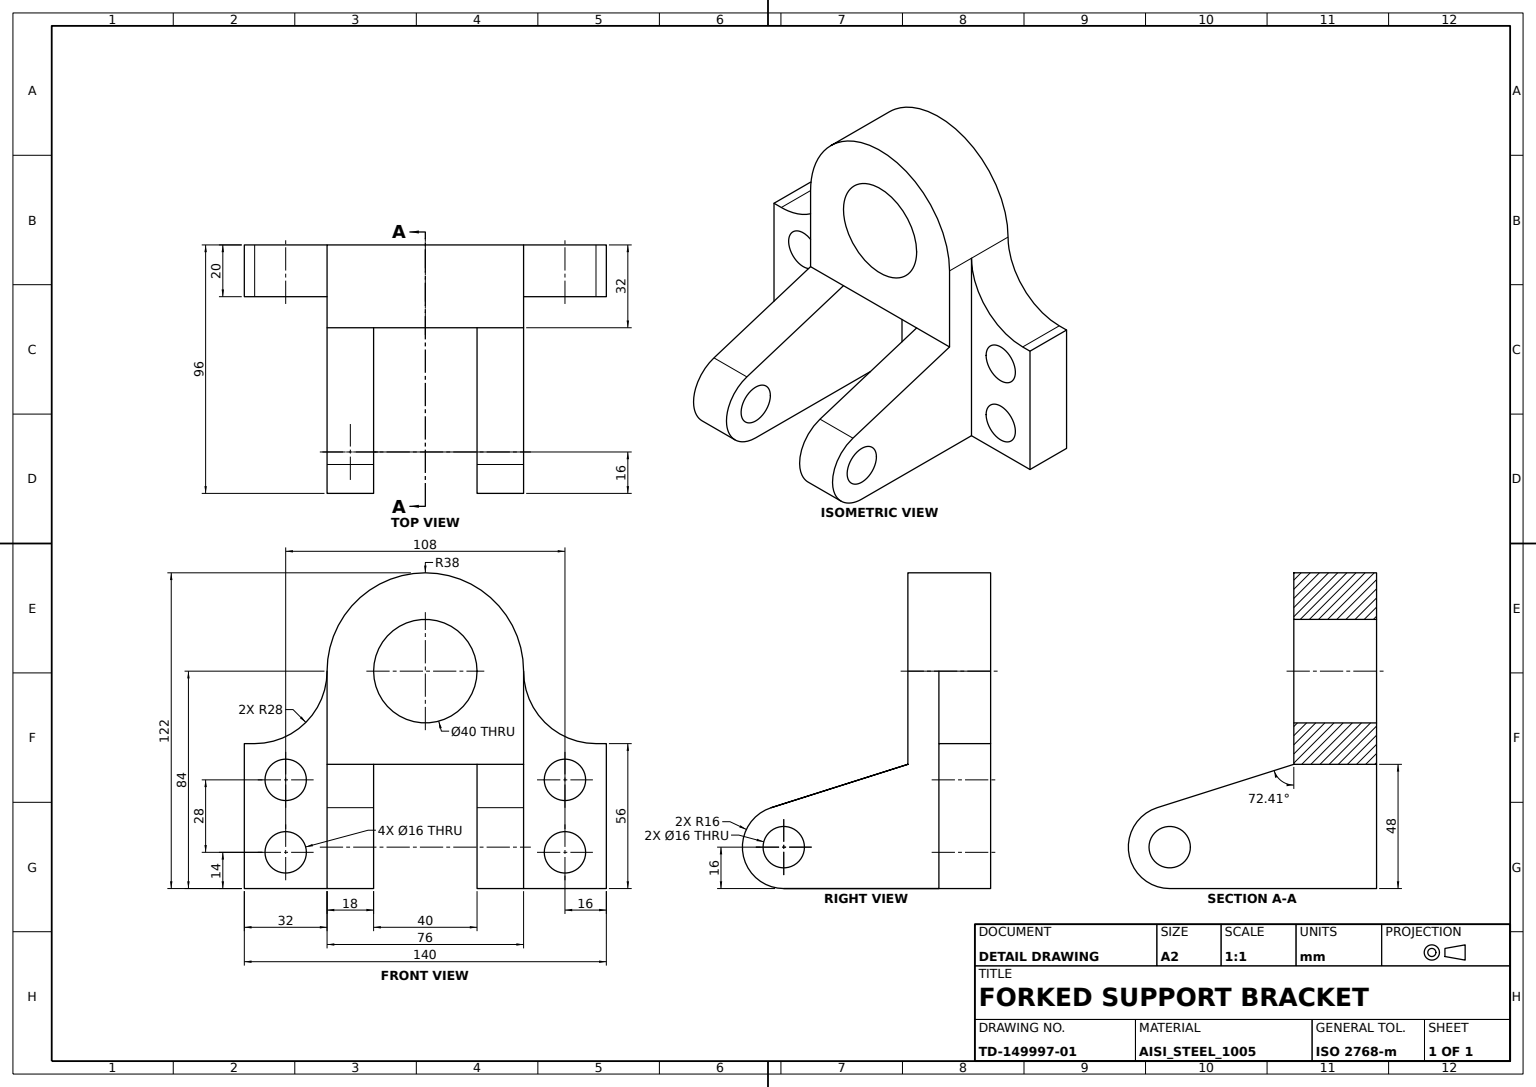
ISO-10303-21;
HEADER;
FILE_DESCRIPTION((''),'2;1');
FILE_NAME('','',(''),(''),'','','');
FILE_SCHEMA(('AUTOMOTIVE_DESIGN'));
ENDSEC;
DATA;
#1=APPLICATION_CONTEXT('');
#2=PRODUCT_CONTEXT('',#1,'mechanical');
#3=PRODUCT('','','',(#2));
#4=PRODUCT_DEFINITION_FORMATION('','',#3);
#5=PRODUCT_DEFINITION_CONTEXT('',#1,'design');
#6=PRODUCT_DEFINITION('','',#4,#5);
#7=PRODUCT_DEFINITION_SHAPE('','',#6);
#8=(LENGTH_UNIT()NAMED_UNIT(*)SI_UNIT(.MILLI.,.METRE.));
#9=(NAMED_UNIT(*)PLANE_ANGLE_UNIT()SI_UNIT($,.RADIAN.));
#10=(NAMED_UNIT(*)SI_UNIT($,.STERADIAN.)SOLID_ANGLE_UNIT());
#11=UNCERTAINTY_MEASURE_WITH_UNIT(LENGTH_MEASURE(0.005),#8,'distance_accuracy_value','');
#12=(GEOMETRIC_REPRESENTATION_CONTEXT(3)GLOBAL_UNCERTAINTY_ASSIGNED_CONTEXT((#11))GLOBAL_UNIT_ASSIGNED_CONTEXT((#8,#9,#10))REPRESENTATION_CONTEXT('',''));
#13=CARTESIAN_POINT('',(-20.,-72.,-68.));
#14=VERTEX_POINT('',#13);
#15=CARTESIAN_POINT('',(-20.,-80.,-68.));
#16=DIRECTION('',(1.,0.,0.));
#17=DIRECTION('',(0.,1.,0.));
#18=AXIS2_PLACEMENT_3D('',#15,#16,#17);
#19=CIRCLE('',#18,8.);
#20=EDGE_CURVE('',#14,#14,#19,.T.);
#21=ORIENTED_EDGE('',*,*,#20,.T.);
#22=EDGE_LOOP('',(#21));
#23=FACE_BOUND('',#22,.T.);
#24=CARTESIAN_POINT('',(-38.,-72.,-68.));
#25=VERTEX_POINT('',#24);
#26=CARTESIAN_POINT('',(-38.,-80.,-68.));
#27=AXIS2_PLACEMENT_3D('',#26,#16,#17);
#28=CIRCLE('',#27,8.);
#29=EDGE_CURVE('',#25,#25,#28,.T.);
#30=ORIENTED_EDGE('',*,*,#29,.F.);
#31=EDGE_LOOP('',(#30));
#32=FACE_BOUND('',#31,.T.);
#33=DIRECTION('',(0.,0.,-1.));
#34=AXIS2_PLACEMENT_3D('',#26,#16,#33);
#35=CYLINDRICAL_SURFACE('',#34,8.);
#36=ADVANCED_FACE('',(#23,#32),#35,.F.);
#37=CARTESIAN_POINT('',(-38.,-84.834712,-52.747932));
#38=VERTEX_POINT('',#37);
#39=CARTESIAN_POINT('',(-20.,-84.834712,-52.747932));
#40=VERTEX_POINT('',#39);
#41=VECTOR('',#16,1000.);
#42=LINE('',#37,#41);
#43=EDGE_CURVE('',#38,#40,#42,.T.);
#44=ORIENTED_EDGE('',*,*,#43,.F.);
#45=CARTESIAN_POINT('',(-38.,-80.,-84.));
#46=VERTEX_POINT('',#45);
#47=DIRECTION('',(-1.,0.,0.));
#48=AXIS2_PLACEMENT_3D('',#26,#47,#17);
#49=CIRCLE('',#48,16.);
#50=EDGE_CURVE('',#46,#38,#49,.T.);
#51=ORIENTED_EDGE('',*,*,#50,.F.);
#52=CARTESIAN_POINT('',(-20.,-80.,-84.));
#53=VERTEX_POINT('',#52);
#54=LINE('',#45,#41);
#55=EDGE_CURVE('',#46,#53,#54,.T.);
#56=ORIENTED_EDGE('',*,*,#55,.T.);
#57=AXIS2_PLACEMENT_3D('',#15,#47,#17);
#58=CIRCLE('',#57,16.);
#59=EDGE_CURVE('',#53,#40,#58,.T.);
#60=ORIENTED_EDGE('',*,*,#59,.T.);
#61=EDGE_LOOP('',(#44,#51,#56,#60));
#62=FACE_BOUND('',#61,.T.);
#63=CYLINDRICAL_SURFACE('',#34,16.);
#64=ADVANCED_FACE('',(#62),#63,.T.);
#65=CARTESIAN_POINT('',(38.,-20.,0.));
#66=VERTEX_POINT('',#65);
#67=CARTESIAN_POINT('',(38.,0.,0.));
#68=VERTEX_POINT('',#67);
#69=VECTOR('',#17,1000.);
#70=LINE('',#65,#69);
#71=EDGE_CURVE('',#66,#68,#70,.T.);
#72=ORIENTED_EDGE('',*,*,#71,.F.);
#73=CARTESIAN_POINT('',(66.,-20.,-28.));
#74=VERTEX_POINT('',#73);
#75=CARTESIAN_POINT('',(66.,-20.,0.));
#76=AXIS2_PLACEMENT_3D('',#75,#17,#47);
#77=CIRCLE('',#76,28.);
#78=EDGE_CURVE('',#74,#66,#77,.T.);
#79=ORIENTED_EDGE('',*,*,#78,.F.);
#80=CARTESIAN_POINT('',(66.,0.,-28.));
#81=VERTEX_POINT('',#80);
#82=LINE('',#73,#69);
#83=EDGE_CURVE('',#74,#81,#82,.T.);
#84=ORIENTED_EDGE('',*,*,#83,.T.);
#85=CARTESIAN_POINT('',(66.,0.,0.));
#86=AXIS2_PLACEMENT_3D('',#85,#17,#47);
#87=CIRCLE('',#86,28.);
#88=EDGE_CURVE('',#81,#68,#87,.T.);
#89=ORIENTED_EDGE('',*,*,#88,.T.);
#90=EDGE_LOOP('',(#72,#79,#84,#89));
#91=FACE_BOUND('',#90,.T.);
#92=DIRECTION('',(0.,0.,1.));
#93=AXIS2_PLACEMENT_3D('',#75,#17,#92);
#94=CYLINDRICAL_SURFACE('',#93,28.);
#95=ADVANCED_FACE('',(#91),#94,.F.);
#96=CARTESIAN_POINT('',(20.,-32.,-36.));
#97=VERTEX_POINT('',#96);
#98=CARTESIAN_POINT('',(20.,-84.834712,-52.747932));
#99=VERTEX_POINT('',#98);
#100=DIRECTION('',(0.,-0.953254219,-0.302169479));
#101=VECTOR('',#100,1000.);
#102=LINE('',#96,#101);
#103=EDGE_CURVE('',#97,#99,#102,.T.);
#104=ORIENTED_EDGE('',*,*,#103,.T.);
#105=CARTESIAN_POINT('',(38.,-84.834712,-52.747932));
#106=VERTEX_POINT('',#105);
#107=VECTOR('',#47,1000.);
#108=LINE('',#105,#107);
#109=EDGE_CURVE('',#106,#99,#108,.T.);
#110=ORIENTED_EDGE('',*,*,#109,.F.);
#111=CARTESIAN_POINT('',(38.,-32.,-36.));
#112=VERTEX_POINT('',#111);
#113=LINE('',#111,#101);
#114=EDGE_CURVE('',#112,#106,#113,.T.);
#115=ORIENTED_EDGE('',*,*,#114,.F.);
#116=LINE('',#111,#107);
#117=EDGE_CURVE('',#112,#97,#116,.T.);
#118=ORIENTED_EDGE('',*,*,#117,.T.);
#119=EDGE_LOOP('',(#104,#110,#115,#118));
#120=FACE_BOUND('',#119,.T.);
#121=DIRECTION('',(0.,0.302169479,-0.953254219));
#122=DIRECTION('',(0.,0.953254219,0.302169479));
#123=AXIS2_PLACEMENT_3D('',#111,#121,#122);
#124=PLANE('',#123);
#125=ADVANCED_FACE('',(#120),#124,.F.);
#126=ORIENTED_EDGE('',*,*,#43,.T.);
#127=CARTESIAN_POINT('',(-20.,-32.,-36.));
#128=VERTEX_POINT('',#127);
#129=VECTOR('',#122,1000.);
#130=LINE('',#39,#129);
#131=EDGE_CURVE('',#40,#128,#130,.T.);
#132=ORIENTED_EDGE('',*,*,#131,.T.);
#133=CARTESIAN_POINT('',(-38.,-32.,-36.));
#134=VERTEX_POINT('',#133);
#135=LINE('',#133,#41);
#136=EDGE_CURVE('',#134,#128,#135,.T.);
#137=ORIENTED_EDGE('',*,*,#136,.F.);
#138=LINE('',#37,#129);
#139=EDGE_CURVE('',#38,#134,#138,.T.);
#140=ORIENTED_EDGE('',*,*,#139,.F.);
#141=EDGE_LOOP('',(#126,#132,#137,#140));
#142=FACE_BOUND('',#141,.T.);
#143=AXIS2_PLACEMENT_3D('',#37,#121,#122);
#144=PLANE('',#143);
#145=ADVANCED_FACE('',(#142),#144,.F.);
#146=CARTESIAN_POINT('',(-70.,-20.,-28.));
#147=VERTEX_POINT('',#146);
#148=CARTESIAN_POINT('',(-70.,0.,-28.));
#149=VERTEX_POINT('',#148);
#150=LINE('',#146,#69);
#151=EDGE_CURVE('',#147,#149,#150,.T.);
#152=ORIENTED_EDGE('',*,*,#151,.T.);
#153=CARTESIAN_POINT('',(-70.,0.,-84.));
#154=VERTEX_POINT('',#153);
#155=VECTOR('',#33,1000.);
#156=LINE('',#148,#155);
#157=EDGE_CURVE('',#149,#154,#156,.T.);
#158=ORIENTED_EDGE('',*,*,#157,.T.);
#159=CARTESIAN_POINT('',(-70.,-20.,-84.));
#160=VERTEX_POINT('',#159);
#161=LINE('',#159,#69);
#162=EDGE_CURVE('',#160,#154,#161,.T.);
#163=ORIENTED_EDGE('',*,*,#162,.F.);
#164=LINE('',#146,#155);
#165=EDGE_CURVE('',#147,#160,#164,.T.);
#166=ORIENTED_EDGE('',*,*,#165,.F.);
#167=EDGE_LOOP('',(#152,#158,#163,#166));
#168=FACE_BOUND('',#167,.T.);
#169=AXIS2_PLACEMENT_3D('',#146,#16,#33);
#170=PLANE('',#169);
#171=ADVANCED_FACE('',(#168),#170,.F.);
#172=CARTESIAN_POINT('',(20.,-32.,0.));
#173=VERTEX_POINT('',#172);
#174=CARTESIAN_POINT('',(0.,-32.,0.));
#175=DIRECTION('',(0.,-1.,0.));
#176=AXIS2_PLACEMENT_3D('',#174,#175,#16);
#177=CIRCLE('',#176,20.);
#178=EDGE_CURVE('',#173,#173,#177,.T.);
#179=ORIENTED_EDGE('',*,*,#178,.T.);
#180=EDGE_LOOP('',(#179));
#181=FACE_BOUND('',#180,.T.);
#182=CARTESIAN_POINT('',(20.,0.,0.));
#183=VERTEX_POINT('',#182);
#184=CARTESIAN_POINT('',(0.,0.,0.));
#185=AXIS2_PLACEMENT_3D('',#184,#175,#16);
#186=CIRCLE('',#185,20.);
#187=EDGE_CURVE('',#183,#183,#186,.T.);
#188=ORIENTED_EDGE('',*,*,#187,.F.);
#189=EDGE_LOOP('',(#188));
#190=FACE_BOUND('',#189,.T.);
#191=AXIS2_PLACEMENT_3D('',#174,#17,#92);
#192=CYLINDRICAL_SURFACE('',#191,20.);
#193=ADVANCED_FACE('',(#181,#190),#192,.F.);
#194=EDGE_CURVE('',#128,#97,#135,.T.);
#195=ORIENTED_EDGE('',*,*,#194,.F.);
#196=CARTESIAN_POINT('',(-20.,0.,-36.));
#197=VERTEX_POINT('',#196);
#198=LINE('',#127,#69);
#199=EDGE_CURVE('',#128,#197,#198,.T.);
#200=ORIENTED_EDGE('',*,*,#199,.T.);
#201=CARTESIAN_POINT('',(20.,0.,-36.));
#202=VERTEX_POINT('',#201);
#203=CARTESIAN_POINT('',(-38.,0.,-36.));
#204=LINE('',#203,#41);
#205=EDGE_CURVE('',#197,#202,#204,.T.);
#206=ORIENTED_EDGE('',*,*,#205,.T.);
#207=VECTOR('',#175,1000.);
#208=LINE('',#201,#207);
#209=EDGE_CURVE('',#202,#97,#208,.T.);
#210=ORIENTED_EDGE('',*,*,#209,.T.);
#211=EDGE_LOOP('',(#195,#200,#206,#210));
#212=FACE_BOUND('',#211,.T.);
#213=AXIS2_PLACEMENT_3D('',#133,#92,#16);
#214=PLANE('',#213);
#215=ADVANCED_FACE('',(#212),#214,.F.);
#216=CARTESIAN_POINT('',(-46.,0.,-70.));
#217=VERTEX_POINT('',#216);
#218=CARTESIAN_POINT('',(-54.,0.,-70.));
#219=AXIS2_PLACEMENT_3D('',#218,#175,#16);
#220=CIRCLE('',#219,8.);
#221=EDGE_CURVE('',#217,#217,#220,.T.);
#222=ORIENTED_EDGE('',*,*,#221,.F.);
#223=EDGE_LOOP('',(#222));
#224=FACE_BOUND('',#223,.T.);
#225=CARTESIAN_POINT('',(-46.,-20.,-70.));
#226=VERTEX_POINT('',#225);
#227=CARTESIAN_POINT('',(-54.,-20.,-70.));
#228=AXIS2_PLACEMENT_3D('',#227,#175,#16);
#229=CIRCLE('',#228,8.);
#230=EDGE_CURVE('',#226,#226,#229,.T.);
#231=ORIENTED_EDGE('',*,*,#230,.T.);
#232=EDGE_LOOP('',(#231));
#233=FACE_BOUND('',#232,.T.);
#234=AXIS2_PLACEMENT_3D('',#227,#17,#92);
#235=CYLINDRICAL_SURFACE('',#234,8.);
#236=ADVANCED_FACE('',(#224,#233),#235,.F.);
#237=CARTESIAN_POINT('',(-38.,-32.,0.));
#238=VERTEX_POINT('',#237);
#239=CARTESIAN_POINT('',(-38.,-20.,0.));
#240=VERTEX_POINT('',#239);
#241=LINE('',#237,#69);
#242=EDGE_CURVE('',#238,#240,#241,.T.);
#243=ORIENTED_EDGE('',*,*,#242,.F.);
#244=CARTESIAN_POINT('',(38.,-32.,0.));
#245=VERTEX_POINT('',#244);
#246=CIRCLE('',#176,38.);
#247=EDGE_CURVE('',#245,#238,#246,.T.);
#248=ORIENTED_EDGE('',*,*,#247,.F.);
#249=LINE('',#244,#69);
#250=EDGE_CURVE('',#245,#66,#249,.T.);
#251=ORIENTED_EDGE('',*,*,#250,.T.);
#252=ORIENTED_EDGE('',*,*,#71,.T.);
#253=CARTESIAN_POINT('',(-38.,0.,0.));
#254=VERTEX_POINT('',#253);
#255=CIRCLE('',#185,38.);
#256=EDGE_CURVE('',#68,#254,#255,.T.);
#257=ORIENTED_EDGE('',*,*,#256,.T.);
#258=LINE('',#239,#69);
#259=EDGE_CURVE('',#240,#254,#258,.T.);
#260=ORIENTED_EDGE('',*,*,#259,.F.);
#261=EDGE_LOOP('',(#243,#248,#251,#252,#257,#260));
#262=FACE_BOUND('',#261,.T.);
#263=CYLINDRICAL_SURFACE('',#191,38.);
#264=ADVANCED_FACE('',(#262),#263,.T.);
#265=CARTESIAN_POINT('',(38.,-72.,-68.));
#266=VERTEX_POINT('',#265);
#267=CARTESIAN_POINT('',(38.,-80.,-68.));
#268=AXIS2_PLACEMENT_3D('',#267,#16,#17);
#269=CIRCLE('',#268,8.);
#270=EDGE_CURVE('',#266,#266,#269,.T.);
#271=ORIENTED_EDGE('',*,*,#270,.F.);
#272=EDGE_LOOP('',(#271));
#273=FACE_BOUND('',#272,.T.);
#274=VECTOR('',#92,1000.);
#275=LINE('',#111,#274);
#276=EDGE_CURVE('',#112,#245,#275,.T.);
#277=ORIENTED_EDGE('',*,*,#276,.F.);
#278=ORIENTED_EDGE('',*,*,#114,.T.);
#279=CARTESIAN_POINT('',(38.,-80.,-84.));
#280=VERTEX_POINT('',#279);
#281=CIRCLE('',#268,16.);
#282=EDGE_CURVE('',#106,#280,#281,.T.);
#283=ORIENTED_EDGE('',*,*,#282,.T.);
#284=CARTESIAN_POINT('',(38.,-20.,-84.));
#285=VERTEX_POINT('',#284);
#286=LINE('',#279,#69);
#287=EDGE_CURVE('',#280,#285,#286,.T.);
#288=ORIENTED_EDGE('',*,*,#287,.T.);
#289=CARTESIAN_POINT('',(38.,-20.,-52.747932));
#290=LINE('',#289,#155);
#291=EDGE_CURVE('',#66,#285,#290,.T.);
#292=ORIENTED_EDGE('',*,*,#291,.F.);
#293=ORIENTED_EDGE('',*,*,#250,.F.);
#294=EDGE_LOOP('',(#277,#278,#283,#288,#292,#293));
#295=FACE_BOUND('',#294,.T.);
#296=AXIS2_PLACEMENT_3D('',#111,#47,#92);
#297=PLANE('',#296);
#298=ADVANCED_FACE('',(#273,#295),#297,.F.);
#299=CARTESIAN_POINT('',(-46.,-20.,-42.));
#300=VERTEX_POINT('',#299);
#301=CARTESIAN_POINT('',(-54.,-20.,-42.));
#302=AXIS2_PLACEMENT_3D('',#301,#175,#16);
#303=CIRCLE('',#302,8.);
#304=EDGE_CURVE('',#300,#300,#303,.T.);
#305=ORIENTED_EDGE('',*,*,#304,.F.);
#306=EDGE_LOOP('',(#305));
#307=FACE_BOUND('',#306,.T.);
#308=ORIENTED_EDGE('',*,*,#230,.F.);
#309=EDGE_LOOP('',(#308));
#310=FACE_BOUND('',#309,.T.);
#311=CARTESIAN_POINT('',(-38.,-20.,-84.));
#312=VERTEX_POINT('',#311);
#313=LINE('',#311,#274);
#314=EDGE_CURVE('',#312,#240,#313,.T.);
#315=ORIENTED_EDGE('',*,*,#314,.T.);
#316=CARTESIAN_POINT('',(-66.,-20.,-28.));
#317=VERTEX_POINT('',#316);
#318=CARTESIAN_POINT('',(-66.,-20.,0.));
#319=AXIS2_PLACEMENT_3D('',#318,#17,#16);
#320=CIRCLE('',#319,28.);
#321=EDGE_CURVE('',#240,#317,#320,.T.);
#322=ORIENTED_EDGE('',*,*,#321,.T.);
#323=LINE('',#316,#107);
#324=EDGE_CURVE('',#317,#147,#323,.T.);
#325=ORIENTED_EDGE('',*,*,#324,.T.);
#326=ORIENTED_EDGE('',*,*,#165,.T.);
#327=LINE('',#159,#41);
#328=EDGE_CURVE('',#160,#312,#327,.T.);
#329=ORIENTED_EDGE('',*,*,#328,.T.);
#330=EDGE_LOOP('',(#315,#322,#325,#326,#329));
#331=FACE_BOUND('',#330,.T.);
#332=AXIS2_PLACEMENT_3D('',#318,#17,#92);
#333=PLANE('',#332);
#334=ADVANCED_FACE('',(#307,#310,#331),#333,.F.);
#335=CARTESIAN_POINT('',(46.,-20.,-70.));
#336=VERTEX_POINT('',#335);
#337=CARTESIAN_POINT('',(54.,-20.,-70.));
#338=AXIS2_PLACEMENT_3D('',#337,#17,#47);
#339=CIRCLE('',#338,8.);
#340=EDGE_CURVE('',#336,#336,#339,.T.);
#341=ORIENTED_EDGE('',*,*,#340,.F.);
#342=EDGE_LOOP('',(#341));
#343=FACE_BOUND('',#342,.T.);
#344=CARTESIAN_POINT('',(46.,0.,-70.));
#345=VERTEX_POINT('',#344);
#346=CARTESIAN_POINT('',(54.,0.,-70.));
#347=AXIS2_PLACEMENT_3D('',#346,#17,#47);
#348=CIRCLE('',#347,8.);
#349=EDGE_CURVE('',#345,#345,#348,.T.);
#350=ORIENTED_EDGE('',*,*,#349,.T.);
#351=EDGE_LOOP('',(#350));
#352=FACE_BOUND('',#351,.T.);
#353=AXIS2_PLACEMENT_3D('',#337,#17,#92);
#354=CYLINDRICAL_SURFACE('',#353,8.);
#355=ADVANCED_FACE('',(#343,#352),#354,.F.);
#356=CARTESIAN_POINT('',(20.,-80.,-84.));
#357=VERTEX_POINT('',#356);
#358=CARTESIAN_POINT('',(20.,-80.,-68.));
#359=AXIS2_PLACEMENT_3D('',#358,#16,#17);
#360=CIRCLE('',#359,16.);
#361=EDGE_CURVE('',#99,#357,#360,.T.);
#362=ORIENTED_EDGE('',*,*,#361,.T.);
#363=LINE('',#279,#107);
#364=EDGE_CURVE('',#280,#357,#363,.T.);
#365=ORIENTED_EDGE('',*,*,#364,.F.);
#366=ORIENTED_EDGE('',*,*,#282,.F.);
#367=ORIENTED_EDGE('',*,*,#109,.T.);
#368=EDGE_LOOP('',(#362,#365,#366,#367));
#369=FACE_BOUND('',#368,.T.);
#370=AXIS2_PLACEMENT_3D('',#267,#47,#92);
#371=CYLINDRICAL_SURFACE('',#370,16.);
#372=ADVANCED_FACE('',(#369),#371,.T.);
#373=CARTESIAN_POINT('',(-46.,0.,-42.));
#374=VERTEX_POINT('',#373);
#375=CARTESIAN_POINT('',(-54.,0.,-42.));
#376=AXIS2_PLACEMENT_3D('',#375,#175,#16);
#377=CIRCLE('',#376,8.);
#378=EDGE_CURVE('',#374,#374,#377,.T.);
#379=ORIENTED_EDGE('',*,*,#378,.F.);
#380=EDGE_LOOP('',(#379));
#381=FACE_BOUND('',#380,.T.);
#382=ORIENTED_EDGE('',*,*,#304,.T.);
#383=EDGE_LOOP('',(#382));
#384=FACE_BOUND('',#383,.T.);
#385=AXIS2_PLACEMENT_3D('',#301,#17,#92);
#386=CYLINDRICAL_SURFACE('',#385,8.);
#387=ADVANCED_FACE('',(#381,#384),#386,.F.);
#388=ORIENTED_EDGE('',*,*,#361,.F.);
#389=ORIENTED_EDGE('',*,*,#103,.F.);
#390=ORIENTED_EDGE('',*,*,#209,.F.);
#391=CARTESIAN_POINT('',(20.,0.,-84.));
#392=VERTEX_POINT('',#391);
#393=LINE('',#391,#274);
#394=EDGE_CURVE('',#392,#202,#393,.T.);
#395=ORIENTED_EDGE('',*,*,#394,.F.);
#396=LINE('',#356,#69);
#397=EDGE_CURVE('',#357,#392,#396,.T.);
#398=ORIENTED_EDGE('',*,*,#397,.F.);
#399=EDGE_LOOP('',(#388,#389,#390,#395,#398));
#400=FACE_BOUND('',#399,.T.);
#401=CARTESIAN_POINT('',(20.,-72.,-68.));
#402=VERTEX_POINT('',#401);
#403=CIRCLE('',#359,8.);
#404=EDGE_CURVE('',#402,#402,#403,.T.);
#405=ORIENTED_EDGE('',*,*,#404,.T.);
#406=EDGE_LOOP('',(#405));
#407=FACE_BOUND('',#406,.T.);
#408=AXIS2_PLACEMENT_3D('',#358,#16,#33);
#409=PLANE('',#408);
#410=ADVANCED_FACE('',(#400,#407),#409,.F.);
#411=CARTESIAN_POINT('',(-20.,0.,-84.));
#412=VERTEX_POINT('',#411);
#413=CARTESIAN_POINT('',(-38.,0.,-84.));
#414=LINE('',#413,#41);
#415=EDGE_CURVE('',#154,#412,#414,.T.);
#416=ORIENTED_EDGE('',*,*,#415,.F.);
#417=ORIENTED_EDGE('',*,*,#157,.F.);
#418=CARTESIAN_POINT('',(-66.,0.,-28.));
#419=VERTEX_POINT('',#418);
#420=LINE('',#418,#107);
#421=EDGE_CURVE('',#419,#149,#420,.T.);
#422=ORIENTED_EDGE('',*,*,#421,.F.);
#423=CARTESIAN_POINT('',(-66.,0.,0.));
#424=AXIS2_PLACEMENT_3D('',#423,#17,#16);
#425=CIRCLE('',#424,28.);
#426=EDGE_CURVE('',#254,#419,#425,.T.);
#427=ORIENTED_EDGE('',*,*,#426,.F.);
#428=ORIENTED_EDGE('',*,*,#256,.F.);
#429=ORIENTED_EDGE('',*,*,#88,.F.);
#430=CARTESIAN_POINT('',(70.,0.,-28.));
#431=VERTEX_POINT('',#430);
#432=LINE('',#430,#107);
#433=EDGE_CURVE('',#431,#81,#432,.T.);
#434=ORIENTED_EDGE('',*,*,#433,.F.);
#435=CARTESIAN_POINT('',(70.,0.,-84.));
#436=VERTEX_POINT('',#435);
#437=LINE('',#435,#274);
#438=EDGE_CURVE('',#436,#431,#437,.T.);
#439=ORIENTED_EDGE('',*,*,#438,.F.);
#440=CARTESIAN_POINT('',(38.,0.,-84.));
#441=LINE('',#440,#107);
#442=EDGE_CURVE('',#436,#392,#441,.T.);
#443=ORIENTED_EDGE('',*,*,#442,.T.);
#444=ORIENTED_EDGE('',*,*,#394,.T.);
#445=ORIENTED_EDGE('',*,*,#205,.F.);
#446=LINE('',#196,#155);
#447=EDGE_CURVE('',#197,#412,#446,.T.);
#448=ORIENTED_EDGE('',*,*,#447,.T.);
#449=EDGE_LOOP('',(#416,#417,#422,#427,#428,#429,#434,#439,#443,#444,#445,#448));
#450=FACE_BOUND('',#449,.T.);
#451=ORIENTED_EDGE('',*,*,#349,.F.);
#452=EDGE_LOOP('',(#451));
#453=FACE_BOUND('',#452,.T.);
#454=CARTESIAN_POINT('',(46.,0.,-42.));
#455=VERTEX_POINT('',#454);
#456=CARTESIAN_POINT('',(54.,0.,-42.));
#457=AXIS2_PLACEMENT_3D('',#456,#17,#47);
#458=CIRCLE('',#457,8.);
#459=EDGE_CURVE('',#455,#455,#458,.T.);
#460=ORIENTED_EDGE('',*,*,#459,.F.);
#461=EDGE_LOOP('',(#460));
#462=FACE_BOUND('',#461,.T.);
#463=ORIENTED_EDGE('',*,*,#221,.T.);
#464=EDGE_LOOP('',(#463));
#465=FACE_BOUND('',#464,.T.);
#466=ORIENTED_EDGE('',*,*,#378,.T.);
#467=EDGE_LOOP('',(#466));
#468=FACE_BOUND('',#467,.T.);
#469=ORIENTED_EDGE('',*,*,#187,.T.);
#470=EDGE_LOOP('',(#469));
#471=FACE_BOUND('',#470,.T.);
#472=AXIS2_PLACEMENT_3D('',#184,#175,#33);
#473=PLANE('',#472);
#474=ADVANCED_FACE('',(#450,#453,#462,#465,#468,#471),#473,.F.);
#475=LINE('',#316,#69);
#476=EDGE_CURVE('',#317,#419,#475,.T.);
#477=ORIENTED_EDGE('',*,*,#476,.T.);
#478=ORIENTED_EDGE('',*,*,#421,.T.);
#479=ORIENTED_EDGE('',*,*,#151,.F.);
#480=ORIENTED_EDGE('',*,*,#324,.F.);
#481=EDGE_LOOP('',(#477,#478,#479,#480));
#482=FACE_BOUND('',#481,.T.);
#483=AXIS2_PLACEMENT_3D('',#316,#33,#47);
#484=PLANE('',#483);
#485=ADVANCED_FACE('',(#482),#484,.F.);
#486=ORIENTED_EDGE('',*,*,#433,.T.);
#487=ORIENTED_EDGE('',*,*,#83,.F.);
#488=CARTESIAN_POINT('',(70.,-20.,-28.));
#489=VERTEX_POINT('',#488);
#490=LINE('',#488,#107);
#491=EDGE_CURVE('',#489,#74,#490,.T.);
#492=ORIENTED_EDGE('',*,*,#491,.F.);
#493=LINE('',#488,#69);
#494=EDGE_CURVE('',#489,#431,#493,.T.);
#495=ORIENTED_EDGE('',*,*,#494,.T.);
#496=EDGE_LOOP('',(#486,#487,#492,#495));
#497=FACE_BOUND('',#496,.T.);
#498=AXIS2_PLACEMENT_3D('',#488,#33,#47);
#499=PLANE('',#498);
#500=ADVANCED_FACE('',(#497),#499,.F.);
#501=CARTESIAN_POINT('',(70.,-20.,-84.));
#502=VERTEX_POINT('',#501);
#503=LINE('',#284,#41);
#504=EDGE_CURVE('',#285,#502,#503,.T.);
#505=ORIENTED_EDGE('',*,*,#504,.F.);
#506=ORIENTED_EDGE('',*,*,#287,.F.);
#507=ORIENTED_EDGE('',*,*,#364,.T.);
#508=ORIENTED_EDGE('',*,*,#397,.T.);
#509=ORIENTED_EDGE('',*,*,#442,.F.);
#510=LINE('',#501,#69);
#511=EDGE_CURVE('',#502,#436,#510,.T.);
#512=ORIENTED_EDGE('',*,*,#511,.F.);
#513=EDGE_LOOP('',(#505,#506,#507,#508,#509,#512));
#514=FACE_BOUND('',#513,.T.);
#515=AXIS2_PLACEMENT_3D('',#279,#92,#175);
#516=PLANE('',#515);
#517=ADVANCED_FACE('',(#514),#516,.F.);
#518=CARTESIAN_POINT('',(46.,-20.,-42.));
#519=VERTEX_POINT('',#518);
#520=CARTESIAN_POINT('',(54.,-20.,-42.));
#521=AXIS2_PLACEMENT_3D('',#520,#17,#47);
#522=CIRCLE('',#521,8.);
#523=EDGE_CURVE('',#519,#519,#522,.T.);
#524=ORIENTED_EDGE('',*,*,#523,.F.);
#525=EDGE_LOOP('',(#524));
#526=FACE_BOUND('',#525,.T.);
#527=ORIENTED_EDGE('',*,*,#459,.T.);
#528=EDGE_LOOP('',(#527));
#529=FACE_BOUND('',#528,.T.);
#530=AXIS2_PLACEMENT_3D('',#520,#17,#92);
#531=CYLINDRICAL_SURFACE('',#530,8.);
#532=ADVANCED_FACE('',(#526,#529),#531,.F.);
#533=ORIENTED_EDGE('',*,*,#415,.T.);
#534=LINE('',#411,#207);
#535=EDGE_CURVE('',#412,#53,#534,.T.);
#536=ORIENTED_EDGE('',*,*,#535,.T.);
#537=ORIENTED_EDGE('',*,*,#55,.F.);
#538=LINE('',#413,#207);
#539=EDGE_CURVE('',#312,#46,#538,.T.);
#540=ORIENTED_EDGE('',*,*,#539,.F.);
#541=ORIENTED_EDGE('',*,*,#328,.F.);
#542=ORIENTED_EDGE('',*,*,#162,.T.);
#543=EDGE_LOOP('',(#533,#536,#537,#540,#541,#542));
#544=FACE_BOUND('',#543,.T.);
#545=AXIS2_PLACEMENT_3D('',#413,#92,#175);
#546=PLANE('',#545);
#547=ADVANCED_FACE('',(#544),#546,.F.);
#548=ORIENTED_EDGE('',*,*,#438,.T.);
#549=ORIENTED_EDGE('',*,*,#494,.F.);
#550=LINE('',#501,#274);
#551=EDGE_CURVE('',#502,#489,#550,.T.);
#552=ORIENTED_EDGE('',*,*,#551,.F.);
#553=ORIENTED_EDGE('',*,*,#511,.T.);
#554=EDGE_LOOP('',(#548,#549,#552,#553));
#555=FACE_BOUND('',#554,.T.);
#556=AXIS2_PLACEMENT_3D('',#501,#47,#92);
#557=PLANE('',#556);
#558=ADVANCED_FACE('',(#555),#557,.F.);
#559=ORIENTED_EDGE('',*,*,#291,.T.);
#560=ORIENTED_EDGE('',*,*,#504,.T.);
#561=ORIENTED_EDGE('',*,*,#551,.T.);
#562=ORIENTED_EDGE('',*,*,#491,.T.);
#563=ORIENTED_EDGE('',*,*,#78,.T.);
#564=EDGE_LOOP('',(#559,#560,#561,#562,#563));
#565=FACE_BOUND('',#564,.T.);
#566=ORIENTED_EDGE('',*,*,#523,.T.);
#567=EDGE_LOOP('',(#566));
#568=FACE_BOUND('',#567,.T.);
#569=ORIENTED_EDGE('',*,*,#340,.T.);
#570=EDGE_LOOP('',(#569));
#571=FACE_BOUND('',#570,.T.);
#572=PLANE('',#93);
#573=ADVANCED_FACE('',(#565,#568,#571),#572,.F.);
#574=ORIENTED_EDGE('',*,*,#539,.T.);
#575=ORIENTED_EDGE('',*,*,#50,.T.);
#576=ORIENTED_EDGE('',*,*,#139,.T.);
#577=LINE('',#237,#155);
#578=EDGE_CURVE('',#238,#134,#577,.T.);
#579=ORIENTED_EDGE('',*,*,#578,.F.);
#580=ORIENTED_EDGE('',*,*,#242,.T.);
#581=ORIENTED_EDGE('',*,*,#314,.F.);
#582=EDGE_LOOP('',(#574,#575,#576,#579,#580,#581));
#583=FACE_BOUND('',#582,.T.);
#584=ORIENTED_EDGE('',*,*,#29,.T.);
#585=EDGE_LOOP('',(#584));
#586=FACE_BOUND('',#585,.T.);
#587=AXIS2_PLACEMENT_3D('',#237,#16,#33);
#588=PLANE('',#587);
#589=ADVANCED_FACE('',(#583,#586),#588,.F.);
#590=ORIENTED_EDGE('',*,*,#247,.T.);
#591=ORIENTED_EDGE('',*,*,#578,.T.);
#592=ORIENTED_EDGE('',*,*,#136,.T.);
#593=ORIENTED_EDGE('',*,*,#194,.T.);
#594=ORIENTED_EDGE('',*,*,#117,.F.);
#595=ORIENTED_EDGE('',*,*,#276,.T.);
#596=EDGE_LOOP('',(#590,#591,#592,#593,#594,#595));
#597=FACE_BOUND('',#596,.T.);
#598=ORIENTED_EDGE('',*,*,#178,.F.);
#599=EDGE_LOOP('',(#598));
#600=FACE_BOUND('',#599,.T.);
#601=AXIS2_PLACEMENT_3D('',#174,#175,#33);
#602=PLANE('',#601);
#603=ADVANCED_FACE('',(#597,#600),#602,.T.);
#604=ORIENTED_EDGE('',*,*,#404,.F.);
#605=EDGE_LOOP('',(#604));
#606=FACE_BOUND('',#605,.T.);
#607=ORIENTED_EDGE('',*,*,#270,.T.);
#608=EDGE_LOOP('',(#607));
#609=FACE_BOUND('',#608,.T.);
#610=CYLINDRICAL_SURFACE('',#370,8.);
#611=ADVANCED_FACE('',(#606,#609),#610,.F.);
#612=ORIENTED_EDGE('',*,*,#476,.F.);
#613=ORIENTED_EDGE('',*,*,#321,.F.);
#614=ORIENTED_EDGE('',*,*,#259,.T.);
#615=ORIENTED_EDGE('',*,*,#426,.T.);
#616=EDGE_LOOP('',(#612,#613,#614,#615));
#617=FACE_BOUND('',#616,.T.);
#618=CYLINDRICAL_SURFACE('',#332,28.);
#619=ADVANCED_FACE('',(#617),#618,.F.);
#620=ORIENTED_EDGE('',*,*,#59,.F.);
#621=ORIENTED_EDGE('',*,*,#535,.F.);
#622=ORIENTED_EDGE('',*,*,#447,.F.);
#623=ORIENTED_EDGE('',*,*,#199,.F.);
#624=ORIENTED_EDGE('',*,*,#131,.F.);
#625=EDGE_LOOP('',(#620,#621,#622,#623,#624));
#626=FACE_BOUND('',#625,.T.);
#627=ORIENTED_EDGE('',*,*,#20,.F.);
#628=EDGE_LOOP('',(#627));
#629=FACE_BOUND('',#628,.T.);
#630=AXIS2_PLACEMENT_3D('',#15,#47,#92);
#631=PLANE('',#630);
#632=ADVANCED_FACE('',(#626,#629),#631,.F.);
#633=CLOSED_SHELL('',(#36,#64,#95,#125,#145,#171,#193,#215,#236,#264,#298,#334,#355,#372,#387,#410,#474,#485,#500,#517,#532,#547,#558,#573,#589,#603,#611,#619,#632));
#634=MANIFOLD_SOLID_BREP('',#633);
#635=ADVANCED_BREP_SHAPE_REPRESENTATION('',(#634),#12);
#636=SHAPE_DEFINITION_REPRESENTATION(#7,#635);
ENDSEC;
END-ISO-10303-21;
